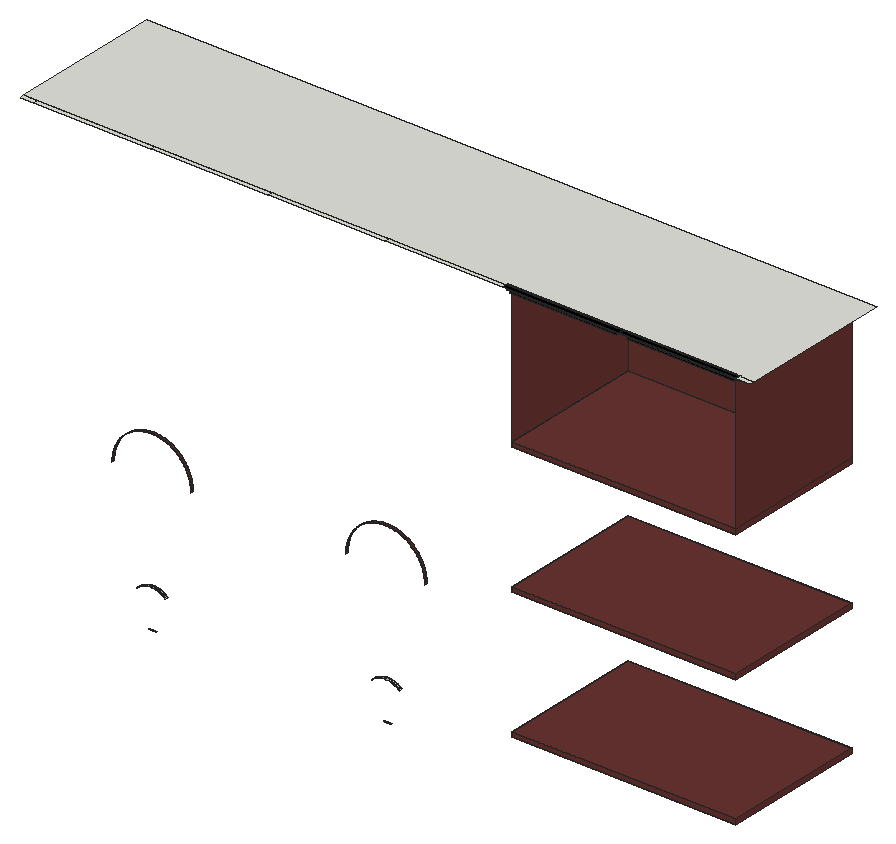
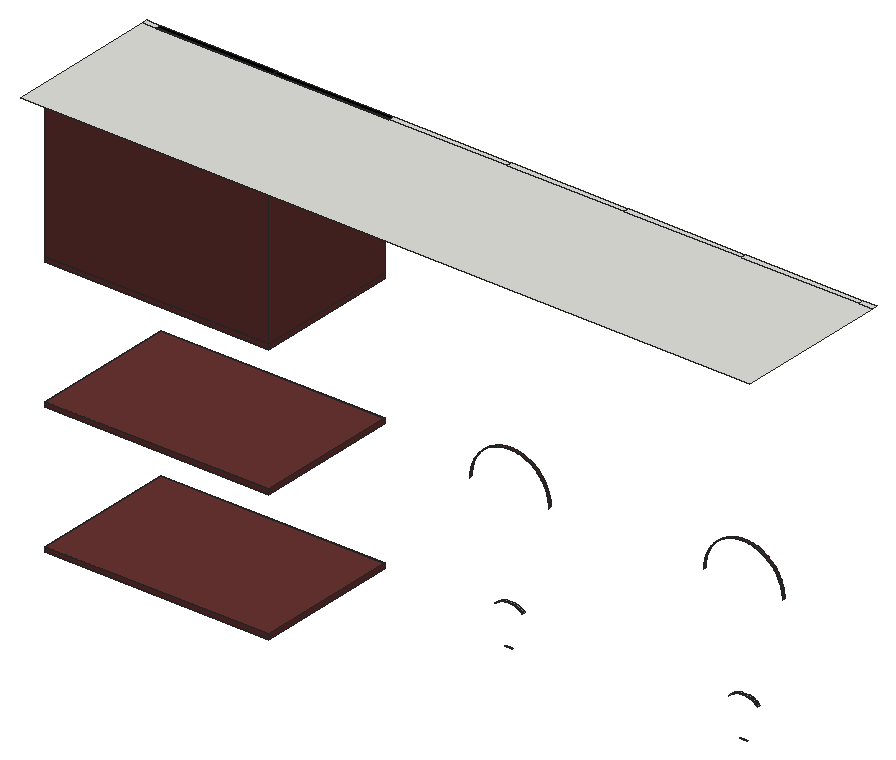
# SketchUp Ruby script. Lengths in millimetres.
U = 1.mm
M = Sketchup.active_model
def pt(a) = Geom::Point3d.new(a.map { |v| v * U })
def face(e, loops, mat)
  f = e.add_face(loops[0].map { |a| pt(a) })
  loops[1..].each { |l| e.add_face(l.map { |a| pt(a) }).erase! }
  f.material = f.back_material = mat if mat
  f
end
# faces: each face lists its corners as indices into pts; further lists are holes
def faces(e, pts, list, mat = nil) = list.each { |f| face(e, (f[0].is_a?(Array) ? f : [f]).map { |l| l.map { |i| pts[i] } }, mat) }
# xy, xz, yz: faces in a plane at the given z, y or x. An outline is a flat list of corners, or four numbers for a rectangle; further outlines are holes
def ring(l) = l.size == 4 ? [[l[0], l[1]], [l[2], l[1]], [l[2], l[3]], [l[0], l[3]]] : l.each_slice(2).to_a
def flat(e, list, mat, &to3) = list.each { |f| face(e, (f[0].is_a?(Array) ? f : [f]).map { |l| ring(l).map { |u, v| to3.(u, v) } }, mat) }
def xy(e, z, list, mat = nil) = flat(e, list, mat) { |x, y| [x, y, z] }
def xz(e, y, list, mat = nil) = flat(e, list, mat) { |x, z| [x, y, z] }
def yz(e, x, list, mat = nil) = flat(e, list, mat) { |y, z| [x, y, z] }
def lines(e, pts, list) = list.each { |a, b| e.add_line(pt(pts[a]), pt(pts[b])) }
# prism: a flat outline (further loops are holes) pulled along v
def prism(e, loops, v, mat = nil)
  f = face(e, loops, mat); d = Geom::Vector3d.new(v.map { |x| x * U })
  f.pushpull(f.normal.samedirection?(d) ? d.length : -d.length)
end
def box(e, o, s, mat = nil) = prism(e, [[o, [o[0] + s[0], o[1], o[2]], [o[0] + s[0], o[1] + s[1], o[2]], [o[0], o[1] + s[1], o[2]]]], [0, 0, s[2]], mat)
def at(x, y, z, deg = 0) = Geom::Transformation.translation(pt([x, y, z])) * Geom::Transformation.rotation(ORIGIN, Z_AXIS, deg.degrees)
def axes(o, x, y, z) = Geom::Transformation.new([*x, 0, *y, 0, *z, 0, *pt(o).to_a, 1])
def part(name) = M.definitions.add(name)
# library, detail: a bought-in or finely detailed component or shape, given as its bounding box
def library(name, o, s) = part(name).tap { |d| box(d.entities, o, s) }
def detail(e, o, s) = box(e.add_group.entities, o, s)
def put(e, d, t, mat = nil) = e.add_instance(d, t).tap { |i| i.material = mat if mat }
def group(e, t, mat = nil) = e.add_group.tap { |g| g.transformation = t; g.material = mat if mat }.entities
root = M.entities
M.materials.add("Uniboard-L17-Ambrette-4K").color = [104, 52, 49]
M.materials.add("Uniboard-L19-Putty-4K").color = [187, 181, 160]
M.materials.add("[Color M09]").color = [0, 0, 0]
c1 = part("Group\#4")
box(c1.entities,[0,0,-18],[863.9,559,18])
xy(root,1371.6,[[604.4,3403.6,618.1,3413.6],[621.1,3403.6,634.7,3413.6],[1510.3,3403.6,1524,3413.6],[1527,3403.6,1540.7,3413.6]],"Uniboard-L19-Putty-4K")
xy(root,2871.6,[[1998,3424.6,2861.9,3983.6]],"Uniboard-L17-Ambrette-4K")
xy(root,2871.6,[[1998,3412.6,2410.4,3421.6],[2449.4,3412.6,2861.9,3421.6]],"[Color M09]")
xy(root,2889.6,[[114.3,3403.6,165.1,3421.6],[168.1,3403.6,618.1,3421.6],[621.1,3403.6,1071,3421.6],[1074,3403.6,1524,3421.6],[1527,3403.6,1977,3421.6],
  [2882.9,3403.6,2933.7,3421.6],[114.3,3421.6,1980,3421.6,1980,3424.6,2879.9,3424.6,2879.9,3421.6,2933.7,3421.6,2933.7,4013.2,114.3,4013.2]])
xy(root,2889.6,[[1980,3403.6,2428.4,3421.6],[2431.4,3403.6,2879.9,3421.6]],"[Color M09]")
xz(root,3413.6,[[617.1,1217.7,618.1,1217.7,618.1,1219.2,604.4,1219.2,609.8,1218.3,612.3,1218,614.7,1217.9],[621.1,1217.7,622,1217.7,624.4,1217.9,626.9,1218,629.3,1218.3,634.7,1219.2,621.1,1219.2],[1523.1,1217.7,1524,1217.7,1524,1219.2,1510.3,1219.2,1513.3,1218.7,1515.8,1218.3,1518.2,1218,1520.6,1217.9],[1527,1217.7,1527.9,1217.7,1530.4,1217.9,1532.8,1218,1535.2,1218.3,1537.7,1218.7,1540.7,1219.2,1527,1219.2],[604.4,1371.6,618.1,1371.6,618.1,1373.1,617.1,1373.1,614.7,1372.9,612.3,1372.8,609.8,1372.5],
  [621.1,1371.6,634.7,1371.6,629.3,1372.5,626.9,1372.8,624.4,1372.9,622,1373.1,621.1,1373.1],[1510.3,1371.6,1524,1371.6,1524,1373.1,1523.1,1373.1,1520.6,1372.9,1518.2,1372.8,1515.8,1372.5,1513.3,1372.1],[1527,1371.6,1540.7,1371.6,1537.7,1372.1,1535.2,1372.5,1532.8,1372.8,1530.4,1372.9,1527.9,1373.1,1527,1373.1]],"Uniboard-L17-Ambrette-4K")
xz(root,3421.6,[[1980,2871.6,2410.4,2889.6],[2449.4,2871.6,2879.9,2889.6]],"[Color M09]")
xz(root,3424.6,[[1980,2871.6,2879.9,2889.6]])
xz(root,3983.6,[[1998,2351.7,2861.9,2871.6]],"Uniboard-L17-Ambrette-4K")
yz(root,468.7,[[3403.6,1752.6,3413.6,1757.4]],"Uniboard-L17-Ambrette-4K")
yz(root,1998,[[3424.6,2351.7,3983.6,2871.6]],"Uniboard-L17-Ambrette-4K")
yz(root,2861.9,[[3424.6,2351.7,3983.6,2871.6]],"Uniboard-L17-Ambrette-4K")
p = [[566.4,3413.6,1352],[564.6,3413.6,1350.3],[564.6,3403.6,1350.3],[566.4,3403.6,1352],[674.5,3413.6,1350.3],[672.8,3413.6,1352],
  [672.8,3403.6,1352],[674.5,3403.6,1350.3],[568.2,3413.6,1353.7],[568.2,3403.6,1353.7],[671,3413.6,1353.7],[671,3403.6,1353.7],
  [1474.1,3413.6,1353.7],[1472.3,3413.6,1352],[1472.3,3403.6,1352],[1474.1,3403.6,1353.7],[1578.7,3413.6,1352],[1576.9,3413.6,1353.7],
  [1576.9,3403.6,1353.7],[1578.7,3403.6,1352],[570,3413.6,1355.3],[570,3403.6,1355.3],[669.1,3413.6,1355.3],[669.1,3403.6,1355.3],
  [1476,3413.6,1355.3],[1476,3403.6,1355.3],[1575,3413.6,1355.3],[1575,3403.6,1355.3],[571.9,3413.6,1356.8],[571.9,3403.6,1356.8],
  [667.2,3413.6,1356.8],[667.2,3403.6,1356.8],[1477.9,3413.6,1356.8],[1477.9,3403.6,1356.8],[1573.1,3413.6,1356.8],[1573.1,3403.6,1356.8],
  [573.9,3413.6,1358.3],[573.9,3403.6,1358.3],[665.2,3413.6,1358.3],[665.2,3403.6,1358.3],[1479.8,3413.6,1358.3],[1479.8,3403.6,1358.3],
  [1571.2,3413.6,1358.3],[1571.2,3403.6,1358.3],[575.9,3413.6,1359.7],[575.9,3403.6,1359.7],[663.2,3413.6,1359.7],[663.2,3403.6,1359.7],
  [1481.8,3413.6,1359.7],[1481.8,3403.6,1359.7],[1569.2,3413.6,1359.7],[1569.2,3403.6,1359.7],[577.9,3413.6,1361],[577.9,3403.6,1361],
  [661.2,3413.6,1361],[661.2,3403.6,1361],[1483.9,3413.6,1361],[1483.9,3403.6,1361],[1567.1,3413.6,1361],[1567.1,3403.6,1361],
  [580,3413.6,1362.3],[580,3403.6,1362.3],[659.1,3413.6,1362.3],[659.1,3403.6,1362.3],[1485.9,3413.6,1362.3],[1485.9,3403.6,1362.3],
  [1565.1,3413.6,1362.3],[1565.1,3403.6,1362.3],[582.1,3413.6,1363.5],[582.1,3403.6,1363.5],[657,3413.6,1363.5],[657,3403.6,1363.5],
  [1488.1,3413.6,1363.5],[1488.1,3403.6,1363.5],[1562.9,3413.6,1363.5],[1562.9,3403.6,1363.5],[584.3,3413.6,1364.6],[584.3,3403.6,1364.6],
  [654.8,3413.6,1364.6],[654.8,3403.6,1364.6],[1490.2,3413.6,1364.6],[1490.2,3403.6,1364.6],[1560.8,3413.6,1364.6],[1560.8,3403.6,1364.6],
  [586.5,3413.6,1365.7],[586.5,3403.6,1365.7],[652.6,3413.6,1365.7],[652.6,3403.6,1365.7],[1492.4,3413.6,1365.7],[1492.4,3403.6,1365.7],
  [1558.6,3413.6,1365.7],[1558.6,3403.6,1365.7],[588.7,3413.6,1366.7],[588.7,3403.6,1366.7],[650.4,3413.6,1366.7],[650.4,3403.6,1366.7],
  [1494.6,3413.6,1366.7],[1494.6,3403.6,1366.7],[1556.4,3413.6,1366.7],[1556.4,3403.6,1366.7],[591,3413.6,1367.6],[591,3403.6,1367.6],
  [648.2,3413.6,1367.6],[648.2,3403.6,1367.6],[1496.9,3413.6,1367.6],[1496.9,3403.6,1367.6],[1554.1,3413.6,1367.6],[1554.1,3403.6,1367.6],
  [593.2,3413.6,1368.5],[593.2,3403.6,1368.5],[645.9,3413.6,1368.5],[645.9,3403.6,1368.5],[1499.2,3413.6,1368.5],[1499.2,3403.6,1368.5],
  [1551.8,3413.6,1368.5],[1551.8,3403.6,1368.5],[595.6,3413.6,1369.3],[595.6,3403.6,1369.3],[643.6,3413.6,1369.3],[643.6,3403.6,1369.3],
  [1501.5,3413.6,1369.3],[1501.5,3403.6,1369.3],[1549.5,3413.6,1369.3],[1549.5,3403.6,1369.3],[597.9,3413.6,1370],[597.9,3403.6,1370],
  [641.2,3413.6,1370],[641.2,3403.6,1370],[1503.8,3413.6,1370],[1503.8,3403.6,1370],[1547.2,3413.6,1370],[1547.2,3403.6,1370],
  [600.2,3413.6,1370.7],[600.2,3403.6,1370.7],[638.9,3413.6,1370.7],[638.9,3403.6,1370.7],[1506.2,3413.6,1370.7],[1506.2,3403.6,1370.7],
  [1544.8,3413.6,1370.7],[1544.8,3403.6,1370.7],[602.6,3413.6,1371.2],[602.6,3403.6,1371.2],[636.5,3413.6,1371.2],[636.5,3403.6,1371.2],
  [1508.6,3413.6,1371.2],[1508.6,3403.6,1371.2],[1542.4,3413.6,1371.2],[1542.4,3403.6,1371.2],[604.4,3413.6,1371.6],[604.4,3403.6,1371.6],
  [634.7,3413.6,1371.6],[634.7,3403.6,1371.6],[1510.3,3413.6,1371.6],[1510.3,3403.6,1371.6],[1540.7,3413.6,1371.6],[1540.7,3403.6,1371.6],
  [773.5,3403.6,1752.6],[773.4,3403.6,1757.4],[773.4,3413.6,1757.4],[773.5,3413.6,1752.6],[1371.7,3403.6,1757.4],[1371.6,3403.6,1752.6],
  [1371.6,3413.6,1752.6],[1371.7,3413.6,1757.4],[1676.4,3403.6,1752.6],[1676.3,3403.6,1757.4],[1676.3,3413.6,1757.4],[1676.4,3413.6,1752.6],
  [469,3403.6,1762.2],[468.7,3403.6,1757.4],[468.7,3413.6,1757.4],[469,3413.6,1762.2],[773.2,3403.6,1762.2],[773.2,3413.6,1762.2],
  [1371.9,3403.6,1762.2],[1371.9,3413.6,1762.2],[1676.1,3403.6,1762.2],[1676.1,3413.6,1762.2],[469.3,3403.6,1766.9],[469.3,3413.6,1766.9],
  [772.8,3403.6,1766.9],[772.8,3413.6,1766.9],[1372.3,3403.6,1766.9],[1372.3,3413.6,1766.9],[1675.7,3403.6,1766.9],[1675.7,3413.6,1766.9],
  [469.9,3403.6,1771.7],[469.9,3413.6,1771.7],[772.3,3403.6,1771.7],[772.3,3413.6,1771.7],[1372.8,3403.6,1771.7],[1372.8,3413.6,1771.7],
  [1675.2,3403.6,1771.7],[1675.2,3413.6,1771.7],[470.5,3403.6,1776.4],[470.5,3413.6,1776.4],[771.6,3403.6,1776.4],[771.6,3413.6,1776.4],
  [1373.5,3403.6,1776.4],[1373.5,3413.6,1776.4],[1674.5,3403.6,1776.4],[1674.5,3413.6,1776.4],[471.4,3403.6,1781.2],[471.4,3413.6,1781.2],
  [770.8,3403.6,1781.2],[770.8,3413.6,1781.2],[1374.3,3403.6,1781.2],[1374.3,3413.6,1781.2],[1673.7,3403.6,1781.2],[1673.7,3413.6,1781.2],
  [472.3,3403.6,1785.8],[472.3,3413.6,1785.8],[769.8,3403.6,1785.8],[769.8,3413.6,1785.8],[1375.3,3403.6,1785.8],[1375.3,3413.6,1785.8],
  [1672.7,3403.6,1785.8],[1672.7,3413.6,1785.8],[473.5,3403.6,1790.5],[473.5,3413.6,1790.5],[768.7,3403.6,1790.5],[768.7,3413.6,1790.5],
  [1376.4,3403.6,1790.5],[1376.4,3413.6,1790.5],[1671.6,3403.6,1790.5],[1671.6,3413.6,1790.5],[474.7,3403.6,1795.1],[474.7,3413.6,1795.1],
  [767.4,3403.6,1795.1],[767.4,3413.6,1795.1],[1377.7,3403.6,1795.1],[1377.7,3413.6,1795.1],[1670.3,3403.6,1795.1],[1670.3,3413.6,1795.1],
  [476.1,3403.6,1799.7],[476.1,3413.6,1799.7],[766,3403.6,1799.7],[766,3413.6,1799.7],[1379.1,3403.6,1799.7],[1379.1,3413.6,1799.7],
  [1668.9,3403.6,1799.7],[1668.9,3413.6,1799.7],[477.7,3403.6,1804.2],[477.7,3413.6,1804.2],[764.5,3403.6,1804.2],[764.5,3413.6,1804.2],
  [1380.6,3403.6,1804.2],[1380.6,3413.6,1804.2],[1667.4,3403.6,1804.2],[1667.4,3413.6,1804.2],[479.4,3403.6,1808.7],[479.4,3413.6,1808.7],
  [762.8,3403.6,1808.7],[762.8,3413.6,1808.7],[1382.3,3403.6,1808.7],[1382.3,3413.6,1808.7],[1665.7,3403.6,1808.7],[1665.7,3413.6,1808.7],
  [481.2,3403.6,1813.1],[481.2,3413.6,1813.1],[760.9,3403.6,1813.1],[760.9,3413.6,1813.1],[1384.1,3403.6,1813.1],[1384.1,3413.6,1813.1],
  [1663.9,3403.6,1813.1],[1663.9,3413.6,1813.1],[483.2,3403.6,1817.5],[483.2,3413.6,1817.5],[759,3403.6,1817.5],[759,3413.6,1817.5],
  [1386.1,3403.6,1817.5],[1386.1,3413.6,1817.5],[1661.9,3403.6,1817.5],[1661.9,3413.6,1817.5],[485.3,3403.6,1821.8],[485.3,3413.6,1821.8],
  [756.9,3403.6,1821.8],[756.9,3413.6,1821.8],[1388.2,3403.6,1821.8],[1388.2,3413.6,1821.8],[1659.8,3403.6,1821.8],[1659.8,3413.6,1821.8],
  [487.5,3403.6,1826],[487.5,3413.6,1826],[754.6,3403.6,1826],[754.6,3413.6,1826],[1390.5,3403.6,1826],[1390.5,3413.6,1826],
  [1657.5,3403.6,1826],[1657.5,3413.6,1826],[489.9,3403.6,1830.2],[489.9,3413.6,1830.2],[752.2,3403.6,1830.2],[752.2,3413.6,1830.2],
  [1392.8,3403.6,1830.2],[1392.8,3413.6,1830.2],[1655.2,3403.6,1830.2],[1655.2,3413.6,1830.2],[492.4,3403.6,1834.3],[492.4,3413.6,1834.3],
  [749.7,3403.6,1834.3],[749.7,3413.6,1834.3],[1395.3,3403.6,1834.3],[1395.3,3413.6,1834.3],[1652.7,3403.6,1834.3],[1652.7,3413.6,1834.3],
  [495,3403.6,1838.3],[495,3413.6,1838.3],[747.1,3403.6,1838.3],[747.1,3413.6,1838.3],[1398,3403.6,1838.3],[1398,3413.6,1838.3],
  [1650,3403.6,1838.3],[1650,3413.6,1838.3],[497.8,3403.6,1842.2],[497.8,3413.6,1842.2],[744.4,3403.6,1842.2],[744.4,3413.6,1842.2],
  [1400.7,3403.6,1842.2],[1400.7,3413.6,1842.2],[1647.3,3403.6,1842.2],[1647.3,3413.6,1842.2],[500.6,3403.6,1846],[500.6,3413.6,1846],
  [741.5,3403.6,1846],[741.5,3413.6,1846],[1403.6,3403.6,1846],[1403.6,3413.6,1846],[1644.4,3403.6,1846],[1644.4,3413.6,1846],
  [503.6,3403.6,1849.7],[503.6,3413.6,1849.7],[738.5,3403.6,1849.7],[738.5,3413.6,1849.7],[1406.6,3403.6,1849.7],[1406.6,3413.6,1849.7],
  [1641.4,3403.6,1849.7],[1641.4,3413.6,1849.7],[506.7,3403.6,1853.4],[506.7,3413.6,1853.4],[735.4,3403.6,1853.4],[735.4,3413.6,1853.4],
  [1409.7,3403.6,1853.4],[1409.7,3413.6,1853.4],[1638.3,3403.6,1853.4],[1638.3,3413.6,1853.4],[510,3403.6,1856.9],[510,3413.6,1856.9],
  [732.2,3403.6,1856.9],[732.2,3413.6,1856.9],[1412.9,3403.6,1856.9],[1412.9,3413.6,1856.9],[1635.1,3403.6,1856.9],[1635.1,3413.6,1856.9],
  [513.3,3403.6,1860.4],[513.3,3413.6,1860.4],[728.8,3403.6,1860.4],[728.8,3413.6,1860.4],[1416.2,3403.6,1860.4],[1416.2,3413.6,1860.4],
  [1631.8,3403.6,1860.4],[1631.8,3413.6,1860.4],[516.7,3403.6,1863.7],[516.7,3413.6,1863.7],[725.4,3403.6,1863.7],[725.4,3413.6,1863.7],
  [1419.7,3403.6,1863.7],[1419.7,3413.6,1863.7],[1628.3,3403.6,1863.7],[1628.3,3413.6,1863.7],[520.3,3403.6,1866.9],[520.3,3413.6,1866.9],
  [721.9,3403.6,1866.9],[721.9,3413.6,1866.9],[1423.2,3403.6,1866.9],[1423.2,3413.6,1866.9],[1624.8,3403.6,1866.9],[1624.8,3413.6,1866.9],
  [523.9,3403.6,1870],[523.9,3413.6,1870],[718.2,3403.6,1870],[718.2,3413.6,1870],[1426.9,3403.6,1870],[1426.9,3413.6,1870],
  [1621.1,3403.6,1870],[1621.1,3413.6,1870],[527.7,3403.6,1873],[527.7,3413.6,1873],[714.5,3403.6,1873],[714.5,3413.6,1873],
  [1430.6,3403.6,1873],[1430.6,3413.6,1873],[1617.4,3403.6,1873],[1617.4,3413.6,1873],[531.5,3403.6,1875.9],[531.5,3413.6,1875.9],
  [710.6,3403.6,1875.9],[710.6,3413.6,1875.9],[1434.4,3403.6,1875.9],[1434.4,3413.6,1875.9],[1613.6,3403.6,1875.9],[1613.6,3413.6,1875.9],
  [535.4,3403.6,1878.6],[535.4,3413.6,1878.6],[706.7,3403.6,1878.6],[706.7,3413.6,1878.6],[1438.3,3403.6,1878.6],[1438.3,3413.6,1878.6],
  [1609.7,3403.6,1878.6],[1609.7,3413.6,1878.6],[539.4,3403.6,1881.3],[539.4,3413.6,1881.3],[702.7,3403.6,1881.3],[702.7,3413.6,1881.3],
  [1442.3,3403.6,1881.3],[1442.3,3413.6,1881.3],[1605.7,3403.6,1881.3],[1605.7,3413.6,1881.3],[543.5,3403.6,1883.8],[543.5,3413.6,1883.8],
  [698.6,3403.6,1883.8],[698.6,3413.6,1883.8],[1446.4,3403.6,1883.8],[1446.4,3413.6,1883.8],[1601.6,3403.6,1883.8],[1601.6,3413.6,1883.8],
  [547.6,3403.6,1886.1],[547.6,3413.6,1886.1],[694.5,3403.6,1886.1],[694.5,3413.6,1886.1],[1450.6,3403.6,1886.1],[1450.6,3413.6,1886.1],
  [1597.4,3403.6,1886.1],[1597.4,3413.6,1886.1],[551.9,3403.6,1888.4],[551.9,3413.6,1888.4],[690.3,3403.6,1888.4],[690.3,3413.6,1888.4],
  [1454.8,3403.6,1888.4],[1454.8,3413.6,1888.4],[1593.2,3403.6,1888.4],[1593.2,3413.6,1888.4],[556.2,3403.6,1890.5],[556.2,3413.6,1890.5],
  [686,3403.6,1890.5],[686,3413.6,1890.5],[1459.1,3403.6,1890.5],[1459.1,3413.6,1890.5],[1588.9,3403.6,1890.5],[1588.9,3413.6,1890.5],
  [560.5,3403.6,1892.5],[560.5,3413.6,1892.5],[681.6,3403.6,1892.5],[681.6,3413.6,1892.5],[1463.5,3403.6,1892.5],[1463.5,3413.6,1892.5],
  [1584.5,3403.6,1892.5],[1584.5,3413.6,1892.5],[565,3403.6,1894.3],[565,3413.6,1894.3],[677.2,3403.6,1894.3],[677.2,3413.6,1894.3],
  [1467.9,3403.6,1894.3],[1467.9,3413.6,1894.3],[1580.1,3403.6,1894.3],[1580.1,3413.6,1894.3],[569.4,3403.6,1896],[569.4,3413.6,1896],
  [672.7,3403.6,1896],[672.7,3413.6,1896],[1472.4,3403.6,1896],[1472.4,3413.6,1896],[1575.6,3403.6,1896],[1575.6,3413.6,1896],
  [574,3403.6,1897.5],[574,3413.6,1897.5],[668.2,3403.6,1897.5],[668.2,3413.6,1897.5],[1476.9,3403.6,1897.5],[1476.9,3413.6,1897.5],
  [1571.1,3403.6,1897.5],[1571.1,3413.6,1897.5],[578.5,3403.6,1898.9],[578.5,3413.6,1898.9],[663.6,3403.6,1898.9],[663.6,3413.6,1898.9],
  [1481.5,3403.6,1898.9],[1481.5,3413.6,1898.9],[1566.5,3403.6,1898.9],[1566.5,3413.6,1898.9],[583.2,3403.6,1900.2],[583.2,3413.6,1900.2],
  [659,3403.6,1900.2],[659,3413.6,1900.2],[1486.1,3403.6,1900.2],[1486.1,3413.6,1900.2],[1561.9,3403.6,1900.2],[1561.9,3413.6,1900.2],
  [587.8,3403.6,1901.3],[587.8,3413.6,1901.3],[654.3,3403.6,1901.3],[654.3,3413.6,1901.3],[1490.8,3403.6,1901.3],[1490.8,3413.6,1901.3],
  [1557.2,3403.6,1901.3],[1557.2,3413.6,1901.3],[592.5,3403.6,1902.3],[592.5,3413.6,1902.3],[649.6,3403.6,1902.3],[649.6,3413.6,1902.3],
  [1495.4,3403.6,1902.3],[1495.4,3413.6,1902.3],[1552.6,3403.6,1902.3],[1552.6,3413.6,1902.3],[597.2,3403.6,1903.1],[597.2,3413.6,1903.1],
  [644.9,3403.6,1903.1],[644.9,3413.6,1903.1],[1500.2,3403.6,1903.1],[1500.2,3413.6,1903.1],[1547.8,3403.6,1903.1],[1547.8,3413.6,1903.1],
  [602,3403.6,1903.8],[602,3413.6,1903.8],[640.2,3403.6,1903.8],[640.2,3413.6,1903.8],[1504.9,3403.6,1903.8],[1504.9,3413.6,1903.8],
  [1543.1,3403.6,1903.8],[1543.1,3413.6,1903.8],[606.7,3403.6,1904.3],[606.7,3413.6,1904.3],[635.4,3403.6,1904.3],[635.4,3413.6,1904.3],
  [1509.7,3403.6,1904.3],[1509.7,3413.6,1904.3],[1538.3,3403.6,1904.3],[1538.3,3413.6,1904.3],[611.5,3403.6,1904.7],[611.5,3413.6,1904.7],
  [630.6,3403.6,1904.7],[630.6,3413.6,1904.7],[1514.4,3403.6,1904.7],[1514.4,3413.6,1904.7],[1533.6,3403.6,1904.7],[1533.6,3413.6,1904.7],
  [616.3,3403.6,1904.9],[616.3,3413.6,1904.9],[625.9,3403.6,1904.9],[625.9,3413.6,1904.9],[1519.2,3403.6,1904.9],[1519.2,3413.6,1904.9],
  [1528.8,3403.6,1904.9],[1528.8,3413.6,1904.9],[618.1,3403.6,1905],[618.1,3413.6,1905],[621.1,3403.6,1905],[621.1,3413.6,1905],
  [1524,3403.6,1905],[1524,3413.6,1905],[1527,3403.6,1905],[1527,3413.6,1905],[1525.5,3413.6,1217.7],[1527,3413.6,1217.7],
  [1524,3413.6,1217.7]]
faces(root,p,[[0,1,2,3],[4,5,6,7],[8,0,3,9],[5,10,11,6],[12,13,14,15],[20,8,9,21],[10,22,23,11],[24,12,15,25],
  [28,20,21,29],[22,30,31,23],[32,24,25,33],[36,28,29,37],[30,38,39,31],[40,32,33,41],[44,36,37,45],[38,46,47,39],
  [48,40,41,49],[52,44,45,53],[46,54,55,47],[56,48,49,57],[60,52,53,61],[54,62,63,55],[64,56,57,65],[68,60,61,69],
  [62,70,71,63],[72,64,65,73],[76,68,69,77],[70,78,79,71],[80,72,73,81],[84,76,77,85],[78,86,87,79],[88,80,81,89],
  [92,84,85,93],[86,94,95,87],[96,88,89,97],[100,92,93,101],[94,102,103,95],[104,96,97,105],[108,100,101,109],[102,110,111,103],
  [112,104,105,113],[116,108,109,117],[110,118,119,111],[120,112,113,121],[124,116,117,125],[118,126,127,119],[128,120,121,129],[132,124,125,133],
  [126,134,135,127],[136,128,129,137],[140,132,133,141],[134,142,143,135],[144,136,137,145],[148,140,141,149],[142,150,151,143],[152,144,145,153]],"Uniboard-L19-Putty-4K")
faces(root,p,[[16,17,18,19],[17,26,27,18],[26,34,35,27],[34,42,43,35],[42,50,51,43],[50,58,59,51],[58,66,67,59],[66,74,75,67],
  [74,82,83,75],[82,90,91,83],[90,98,99,91],[98,106,107,99],[106,114,115,107],[114,122,123,115],[122,130,131,123],[130,138,139,131],
  [138,146,147,139],[146,154,155,147]])
faces(root,p,[[156,157,158,159],[160,161,162,163],[164,165,166,167],[168,169,170,171],[157,172,173,158],[174,160,163,175],[165,176,177,166],[178,168,171,179],
  [172,180,181,173],[182,174,175,183],[176,184,185,177],[186,178,179,187],[180,188,189,181],[190,182,183,191],[184,192,193,185],[194,186,187,195],
  [188,196,197,189],[198,190,191,199],[192,200,201,193],[202,194,195,203],[196,204,205,197],[206,198,199,207],[200,208,209,201],[210,202,203,211],
  [204,212,213,205],[214,206,207,215],[208,216,217,209],[218,210,211,219],[212,220,221,213],[222,214,215,223],[216,224,225,217],[226,218,219,227],
  [220,228,229,221],[230,222,223,231],[224,232,233,225],[234,226,227,235],[228,236,237,229],[238,230,231,239],[232,240,241,233],[242,234,235,243],
  [236,244,245,237],[246,238,239,247],[240,248,249,241],[250,242,243,251],[244,252,253,245],[254,246,247,255],[248,256,257,249],[258,250,251,259],
  [252,260,261,253],[262,254,255,263],[256,264,265,257],[266,258,259,267],[260,268,269,261],[270,262,263,271],[264,272,273,265],[274,266,267,275],
  [268,276,277,269],[278,270,271,279],[272,280,281,273],[282,274,275,283],[276,284,285,277],[286,278,279,287],[280,288,289,281],[290,282,283,291],
  [284,292,293,285],[294,286,287,295],[288,296,297,289],[298,290,291,299],[292,300,301,293],[302,294,295,303],[296,304,305,297],[306,298,299,307],
  [300,308,309,301],[310,302,303,311],[304,312,313,305],[314,306,307,315],[308,316,317,309],[318,310,311,319],[312,320,321,313],[322,314,315,323],
  [316,324,325,317],[326,318,319,327],[320,328,329,321],[330,322,323,331],[324,332,333,325],[334,326,327,335],[328,336,337,329],[338,330,331,339],
  [332,340,341,333],[342,334,335,343],[336,344,345,337],[346,338,339,347],[340,348,349,341],[350,342,343,351],[344,352,353,345],[354,346,347,355],
  [348,356,357,349],[358,350,351,359],[352,360,361,353],[362,354,355,363],[356,364,365,357],[366,358,359,367],[360,368,369,361],[370,362,363,371],
  [364,372,373,365],[374,366,367,375],[368,376,377,369],[378,370,371,379],[372,380,381,373],[382,374,375,383],[376,384,385,377],[386,378,379,387],
  [380,388,389,381],[390,382,383,391],[384,392,393,385],[394,386,387,395],[388,396,397,389],[398,390,391,399],[392,400,401,393],[402,394,395,403],
  [396,404,405,397],[406,398,399,407],[400,408,409,401],[410,402,403,411],[404,412,413,405],[414,406,407,415],[408,416,417,409],[418,410,411,419],
  [412,420,421,413],[422,414,415,423],[416,424,425,417],[426,418,419,427],[420,428,429,421],[430,422,423,431],[424,432,433,425],[434,426,427,435],
  [428,436,437,429],[438,430,431,439],[432,440,441,433],[442,434,435,443],[436,444,445,437],[446,438,439,447],[440,448,449,441],[450,442,443,451],
  [444,452,453,445],[454,446,447,455],[448,456,457,449],[458,450,451,459],[452,460,461,453],[462,454,455,463],[456,464,465,457],[466,458,459,467],
  [460,468,469,461],[470,462,463,471],[464,472,473,465],[474,466,467,475],[468,476,477,469],[478,470,471,479],[472,480,481,473],[482,474,475,483],
  [476,484,485,477],[486,478,479,487],[480,488,489,481],[490,482,483,491],[484,492,493,485],[494,486,487,495],[488,496,497,489],[498,490,491,499],
  [492,500,501,493],[502,494,495,503],[496,504,505,497],[506,498,499,507],[500,508,509,501],[510,502,503,511],[504,512,513,505],[514,506,507,515],
  [508,516,517,509],[518,510,511,519],[512,520,521,513],[522,514,515,523],[516,524,525,517],[526,518,519,527],[520,528,529,521],[530,522,523,531],
  [524,532,533,525],[534,526,527,535],[528,536,537,529],[538,530,531,539],[532,540,541,533],[542,534,535,543],[536,544,545,537],[546,538,539,547],
  [540,548,549,541],[550,542,543,551],[544,552,553,545],[554,546,547,555],[548,556,557,549],[558,550,551,559],[552,560,561,553]],"Uniboard-L17-Ambrette-4K")
lines(root,p,[[562,563],[564,562]])
put(root,c1,at(1998,3424.6,1347.8),"Uniboard-L17-Ambrette-4K")
put(root,c1,at(1998,3424.6,1849.8),"Uniboard-L17-Ambrette-4K")
put(root,c1,at(1998,3424.6,2351.7),"Uniboard-L17-Ambrette-4K")
